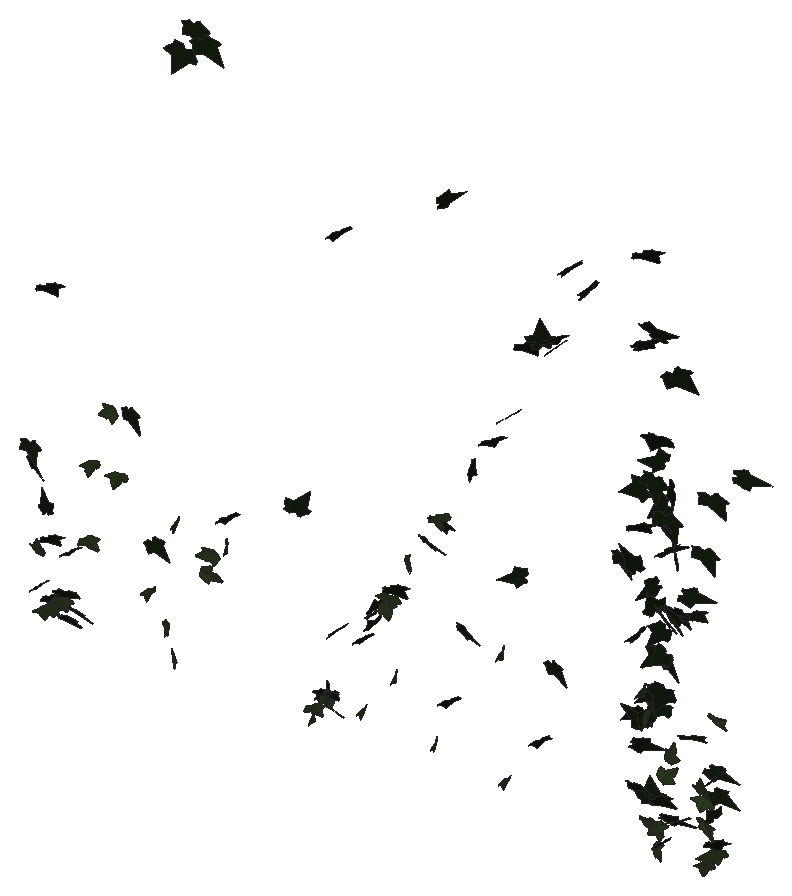
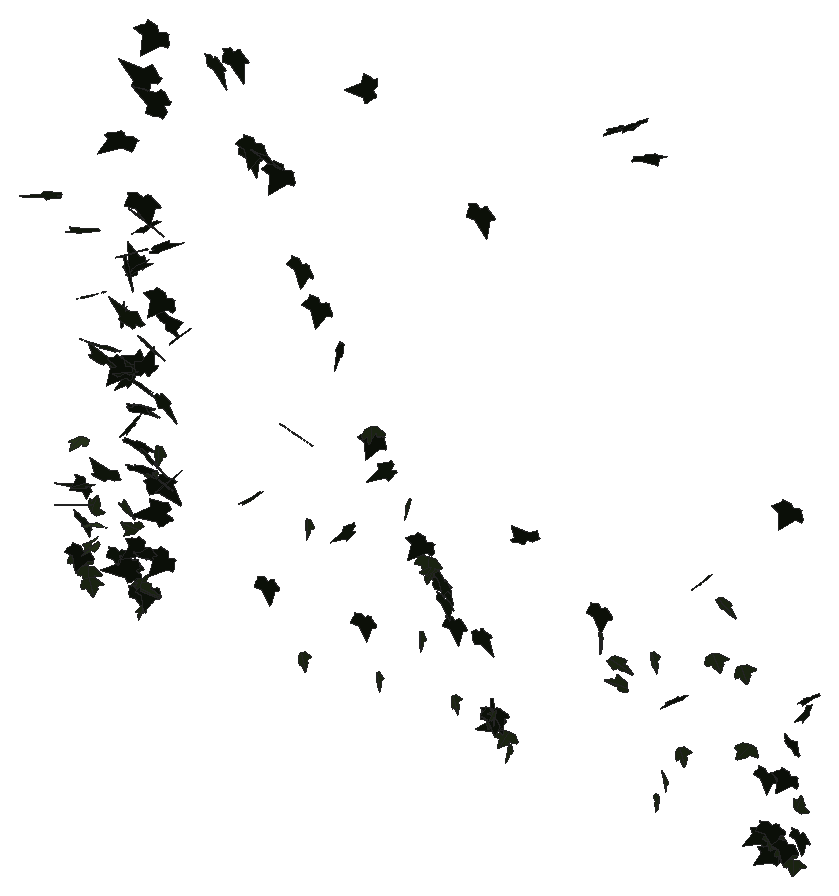
# SketchUp Ruby script. Lengths in inches.
U = 1.inch
M = Sketchup.active_model
def pt(a) = Geom::Point3d.new(a.map { |v| v * U })
def face(e, loops, mat)
  f = e.add_face(loops[0].map { |a| pt(a) })
  loops[1..].each { |l| e.add_face(l.map { |a| pt(a) }).erase! }
  f.material = f.back_material = mat if mat
  f
end
# faces: each face lists its corners as indices into pts; further lists are holes
def faces(e, pts, list, mat = nil) = list.each { |f| face(e, (f[0].is_a?(Array) ? f : [f]).map { |l| l.map { |i| pts[i] } }, mat) }
# xy, xz, yz: faces in a plane at the given z, y or x. An outline is a flat list of corners, or four numbers for a rectangle; further outlines are holes
def ring(l) = l.size == 4 ? [[l[0], l[1]], [l[2], l[1]], [l[2], l[3]], [l[0], l[3]]] : l.each_slice(2).to_a
def flat(e, list, mat, &to3) = list.each { |f| face(e, (f[0].is_a?(Array) ? f : [f]).map { |l| ring(l).map { |u, v| to3.(u, v) } }, mat) }
def xy(e, z, list, mat = nil) = flat(e, list, mat) { |x, y| [x, y, z] }
def xz(e, y, list, mat = nil) = flat(e, list, mat) { |x, z| [x, y, z] }
def yz(e, x, list, mat = nil) = flat(e, list, mat) { |y, z| [x, y, z] }
def lines(e, pts, list) = list.each { |a, b| e.add_line(pt(pts[a]), pt(pts[b])) }
# prism: a flat outline (further loops are holes) pulled along v
def prism(e, loops, v, mat = nil)
  f = face(e, loops, mat); d = Geom::Vector3d.new(v.map { |x| x * U })
  f.pushpull(f.normal.samedirection?(d) ? d.length : -d.length)
end
def box(e, o, s, mat = nil) = prism(e, [[o, [o[0] + s[0], o[1], o[2]], [o[0] + s[0], o[1] + s[1], o[2]], [o[0], o[1] + s[1], o[2]]]], [0, 0, s[2]], mat)
def at(x, y, z, deg = 0) = Geom::Transformation.translation(pt([x, y, z])) * Geom::Transformation.rotation(ORIGIN, Z_AXIS, deg.degrees)
def axes(o, x, y, z) = Geom::Transformation.new([*x, 0, *y, 0, *z, 0, *pt(o).to_a, 1])
def part(name) = M.definitions.add(name)
# library, detail: a bought-in or finely detailed component or shape, given as its bounding box
def library(name, o, s) = part(name).tap { |d| box(d.entities, o, s) }
def detail(e, o, s) = box(e.add_group.entities, o, s)
def put(e, d, t, mat = nil) = e.add_instance(d, t).tap { |i| i.material = mat if mat }
def group(e, t, mat = nil) = e.add_group.tap { |g| g.transformation = t; g.material = mat if mat }.entities
root = M.entities
M.materials.add("1026 AP 7946 SUNNY SIDE UP").color = [254, 231, 186]
M.materials.add("efeu1").color = [18, 25, 13]
M.materials.add("efeu2").color = [43, 57, 29]
c1 = part("ivyleaf_9")
p = [[1.54,2.16,1.25],[1.36,2.04,1.19],[-0.21,0.99,0.68],[-0.71,1.11,0.82],[-0.85,0.86,0.67],[-0.8,0.17,0.21],
  [-0.9,-0.01,0.1],[-0.67,-0.16,-0.02],[-0.08,-0.08,-0.05],[-0.03,-0.6,-0.4],[0.65,-0.88,-0.66],[0.83,-0.6,-0.49],
  [1.29,-0.42,-0.43],[1.8125,-0.07,-0.26],[1.21,0.44,0.15]]
faces(c1.entities,p,[[0,1,2,3,4,5,6,7,8,9,10,11,12,13,14]],"efeu1")
c2 = part("ivyleaf_10")
p = [[0,0.5,-0.03],[-0.0625,2.02,-0.43],[-0.19,2.01,-0.46],[-0.54,1.05,-0.29],[-0.52,0.625,-0.18],[-0.83,0.76,-0.28],
  [-1.16,0.64,-0.33],[-1.15,0.33,-0.24],[-0.77,-0.39,0.02],[-0.3,-0.51,0.16],[0.04,-0.48,0.23],[-0.02,2.01,-0.4375],
  [-0.06,2.01,-0.43],[0.04,-0.49,0.23],[0.67,-0.49,0.14],[1.38,0.36,-0.2],[1.375,0.51,-0.24],[0.81,0.65,-0.19],
  [0.62,0.59,-0.15],[0.6,1.09,-0.28],[0.5,1.23,-0.31]]
faces(c2.entities,p,[[0,1,2,3,4,5,6,7,8,9,10],[11,12,0,13,14,15,16,17,18,19,20]],"efeu2")
put(root,c1,axes([95.23,213.03,300.93],[-0.00357,-0.35074,-0.05937],[-0.00807,0.05091,-0.37476],[0.60158,-0.0014,-0.00538]),"1026 AP 7946 SUNNY SIDE UP")
put(root,c1,axes([95.375,212.96,300.02],[0.35506,-0.28,-0.0458],[-0.08733,0.01017,-0.37215],[0.47192,0.21255,-0.0344]),"1026 AP 7946 SUNNY SIDE UP")
put(root,c2,axes([95.79,213.17,294.47],[-0.49841,0.14012,-0.04801],[-0.04733,0.04941,0.34726],[0.2462,0.29316,-0.03043]),"1026 AP 7946 SUNNY SIDE UP")
put(root,c1,axes([96.05,212.75,292.63],[0.02986,0.32766,0.05959],[0.00064,0.05144,-0.35056],[-0.56301,0.01744,0.00277]),"1026 AP 7946 SUNNY SIDE UP")
put(root,c2,axes([96.24,213.05,291.09],[-0.39048,-0.21835,-0.01454],[0.02991,-0.00298,-0.33924],[0.3699,-0.23026,0.01208]),"1026 AP 7946 SUNNY SIDE UP")
put(root,c1,axes([96.5625,212.75,297.47],[0.19322,-0.04509,0.34792],[-0.15962,0.32567,0.08803],[-0.53463,-0.11353,0.09946]),"1026 AP 7946 SUNNY SIDE UP")
put(root,c1,axes([96.58,213.09,291.97],[0.30177,0.26789,-0.03101],[-0.00319,-0.03764,-0.34411],[-0.45807,0.17674,-0.01803]),"1026 AP 7946 SUNNY SIDE UP")
put(root,c1,axes([96.59,212.74,311.18],[0.44809,0.28118,0.02195],[0.0544,-0.00705,-0.41188],[-0.47507,0.26441,-0.02646]),"1026 AP 7946 SUNNY SIDE UP")
put(root,c2,axes([96.82,213.03,291.51],[-0.41117,-0.21127,-0.01285],[0.0413,-0.01387,-0.34312],[0.35661,-0.24199,0.02492]),"1026 AP 7946 SUNNY SIDE UP")
put(root,c1,axes([96.7,212.79,295.78],[0.40006,0.24658,0.05647],[0.08086,0.0229,-0.36431],[-0.41922,0.23973,-0.01637]),"1026 AP 7946 SUNNY SIDE UP")
put(root,c1,axes([97.14,212.86,291.79],[0.255,-0.06268,-0.30217],[-0.43607,0.11502,-0.17261],[0.22227,0.29756,0.00803]),"1026 AP 7946 SUNNY SIDE UP")
put(root,c2,axes([97.4,213.03,292.11],[-0.48203,-0.15261,-0.08488],[0.14499,-0.00375,-0.34998],[0.23021,-0.31719,0.0427]),"1026 AP 7946 SUNNY SIDE UP")
put(root,c1,axes([97.64,213.05,292.67],[0.31298,0.23347,-0.18068],[-0.20887,-0.11841,-0.31601],[-0.41029,0.23838,0.02305]),"1026 AP 7946 SUNNY SIDE UP")
put(root,c1,axes([97.52,213.03,291.13],[0.53819,0.0485,0.03464],[0.04617,0.03125,-0.34174],[-0.08686,0.31709,0.03295]),"1026 AP 7946 SUNNY SIDE UP")
put(root,c1,axes([98.125,212.8,295.44],[0.11966,0.33328,0.0627],[-0.00067,0.05547,-0.36371],[-0.5732,0.06951,0.01351]),"1026 AP 7946 SUNNY SIDE UP")
put(root,c1,axes([98.24,212.92,291.89],[0.55206,-0.05466,0.00803],[0.02378,0.04489,-0.36262],[0.08357,0.34831,0.05012]),"1026 AP 7946 SUNNY SIDE UP")
put(root,c2,axes([99.45,213.125,301.125],[-0.25583,-0.33417,0.09549],[0.01008,-0.10733,-0.37988],[0.546,-0.15459,0.05176]),"1026 AP 7946 SUNNY SIDE UP")
put(root,c2,axes([99.3,212.87,296.55],[-0.4094,-0.19196,-0.19442],[0.28625,0.06582,-0.32923],[0.31019,-0.3141,0.04722]),"1026 AP 7946 SUNNY SIDE UP")
put(root,c2,axes([100.64,213.28,304.64],[0.35432,-0.1591,-0.29218],[-0.40232,0.12445,-0.28151],[0.31358,0.33943,-0.03105]),"1026 AP 7946 SUNNY SIDE UP")
put(root,c2,axes([101.34,213.03,301.08],[-0.38148,-0.27016,0.12577],[-0.0591,-0.1304,-0.37036],[0.4634,-0.23903,0.0563]),"1026 AP 7946 SUNNY SIDE UP")
put(root,c1,axes([102.03,213.05,305.25],[0.18444,-0.37691,-0.04427],[-0.01339,0.04011,-0.4064],[0.59596,0.11754,0.00457]),"1026 AP 7946 SUNNY SIDE UP")
put(root,c2,axes([103.52,212.97,294.88],[-0.10461,-0.35823,0.02798],[-0.00227,-0.02942,-0.3755],[0.56514,-0.06643,0.00367]),"1026 AP 7946 SUNNY SIDE UP")
put(root,c1,axes([103.71,212.95,297.9],[0.17457,-0.29747,-0.21032],[0.02539,0.21579,-0.31624],[0.56524,0.08218,0.07916]),"1026 AP 7946 SUNNY SIDE UP")
put(root,c2,axes([104.65,212.95,293.1],[0.33264,-0.28479,-0.06698],[0.0119,0.08364,-0.36056],[0.45861,0.20439,0.05794]),"1026 AP 7946 SUNNY SIDE UP")
put(root,c2,axes([105.1,212.9,291.56],[-0.31441,0.29117,-0.04315],[-0.03658,-0.06809,-0.35946],[-0.46148,-0.19298,0.05789]),"1026 AP 7946 SUNNY SIDE UP")
put(root,c2,axes([105.3,212.97,299.71],[0.09906,-0.37566,-0.0326],[-0.00046,0.02987,-0.39221],[0.59251,0.06283,0.00514]),"1026 AP 7946 SUNNY SIDE UP")
put(root,c1,axes([105.63,213.23,328.52],[-0.45543,-0.35945,0.04426],[-0.01019,-0.05248,-0.47501],[0.56953,-0.28838,0.0269]),"1026 AP 7946 SUNNY SIDE UP")
put(root,c1,axes([106.27,213.29,330.24],[0.02494,-0.45731,-0.10528],[0.08561,0.10078,-0.46719],[0.73093,0.0038,0.05831]),"1026 AP 7946 SUNNY SIDE UP")
put(root,c1,axes([107.09,213.05,329.66],[0.0926,-0.40174,-0.24082],[0.19337,0.23852,-0.39283],[0.70295,-0.01269,0.13978]),"1026 AP 7946 SUNNY SIDE UP")
put(root,c2,axes([107.83,212.91,298.5625],[0.30268,-0.02002,-0.3376],[-0.5101,0.04598,-0.199],[0.07825,0.37717,0.00859]),"1026 AP 7946 SUNNY SIDE UP")
put(root,c2,axes([107.32,212.875,297.33],[0.07018,0.04826,0.38191],[0.57347,0.07517,-0.05492],[-0.12722,0.36547,-0.03687]),"1026 AP 7946 SUNNY SIDE UP")
put(root,c1,axes([108.75,212.9,301.2],[0.11336,0.38252,0.00033],[0.00233,-0.00216,-0.40101],[-0.60147,0.07209,-0.00149]),"1026 AP 7946 SUNNY SIDE UP")
put(root,c2,axes([108.82,212.82,299.59],[0.19604,-0.33424,-0.14877],[0.01982,0.15455,-0.36117],[0.57099,0.10939,0.06361]),"1026 AP 7946 SUNNY SIDE UP")
put(root,c1,axes([113.66,212.71,303.45],[-0.32406,-0.02014,0.35571],[0.51548,0.11716,0.20924],[-0.17392,0.38477,-0.04263]),"1026 AP 7946 SUNNY SIDE UP")
put(root,c2,axes([114.67,212.85,291.18],[0.0971,-0.28199,-0.21864],[0.03921,0.21682,-0.29024],[0.55206,0.0342,0.05907]),"1026 AP 7946 SUNNY SIDE UP")
put(root,c2,axes([114.82,212.82,291.8125],[-0.36896,-0.22627,-0.15802],[0.20942,0.07997,-0.33376],[0.37406,-0.26796,0.031]),"1026 AP 7946 SUNNY SIDE UP")
put(root,c1,axes([115.63,212.88,292.9],[0.24167,0.2189,-0.25071],[-0.24008,-0.19142,-0.27643],[-0.4569,0.21636,0.01264]),"1026 AP 7946 SUNNY SIDE UP")
put(root,c1,axes([115.58,212.84,292.79],[0.14638,0.35072,-0.0142],[-0.006,-0.01531,-0.37391],[-0.552,0.09317,0.0003]),"1026 AP 7946 SUNNY SIDE UP")
put(root,c2,axes([115.59,212.85,292.84],[-0.11215,0.3515,0.01797],[-0.085,0.00463,-0.36556],[-0.54666,-0.07283,0.05315]),"1026 AP 7946 SUNNY SIDE UP")
put(root,c1,axes([115.84,212.77,293.3],[0.16952,-0.09094,-0.34698],[-0.49821,0.12074,-0.13757],[0.2277,0.33187,-0.04269]),"1026 AP 7946 SUNNY SIDE UP")
put(root,c2,axes([115.58,212.85,292.66],[0.24726,0.29598,0.14444],[0.01136,0.15055,-0.33894],[-0.51373,0.14579,0.06203]),"1026 AP 7946 SUNNY SIDE UP")
put(root,c1,axes([115.31,212.87,292.26],[0.48861,-0.17513,0.05272],[0.11765,0.02805,-0.36197],[0.26213,0.31384,0.06419]),"1026 AP 7946 SUNNY SIDE UP")
put(root,c1,axes([116.48,212.89,297.1],[-0.16077,0.33809,-0.12939],[0.01209,-0.13046,-0.36345],[-0.56804,-0.09847,0.02888]),"1026 AP 7946 SUNNY SIDE UP")
put(root,c1,axes([116.51,212.83,321.45],[0.03351,0.44655,-0.06141],[-0.00041,-0.06221,-0.46091],[-0.70892,0.02114,-0.00264]),"1026 AP 7946 SUNNY SIDE UP")
put(root,c1,axes([118.16,212.81,297.16],[0.03937,0.37771,-0.00849],[0.00029,-0.01042,-0.39003],[-0.59413,0.02503,-0.00075]),"1026 AP 7946 SUNNY SIDE UP")
put(root,c2,axes([118.11,212.9375,292.76],[0.03919,-0.35756,-0.00565],[0.00814,0.00382,-0.36918],[0.56219,0.02487,0.00574]),"1026 AP 7946 SUNNY SIDE UP")
put(root,c1,axes([118.82,212.83,298.2],[-0.06508,0.33985,0.17693],[-0.06461,0.16581,-0.35121],[-0.59387,-0.05528,0.01882]),"1026 AP 7946 SUNNY SIDE UP")
put(root,c1,axes([118.9375,212.77,299.23],[0.04365,0.2671,0.28509],[-0.03407,0.27659,-0.27267],[-0.60209,0.00372,0.0361]),"1026 AP 7946 SUNNY SIDE UP")
put(root,c1,axes([119.13,212.78,299.11],[-0.17113,0.36333,-0.02991],[-0.04093,-0.04011,-0.38917],[-0.57193,-0.10585,0.0368]),"1026 AP 7946 SUNNY SIDE UP")
put(root,c2,axes([119.63,212.82,299.62],[0.19033,0.35589,0.09671],[0.00542,0.09561,-0.38572],[-0.57791,0.11811,0.02824]),"1026 AP 7946 SUNNY SIDE UP")
put(root,c2,axes([119.81,212.97,300.17],[-0.58691,-0.09079,0.01008],[-0.00338,-0.03459,-0.39447],[0.14364,-0.37179,0.03191]),"1026 AP 7946 SUNNY SIDE UP")
put(root,c2,axes([120.31,212.87,295.63],[0.08062,-0.32197,-0.17951],[0.00294,0.17434,-0.33379],[0.57428,0.04431,0.02691]),"1026 AP 7946 SUNNY SIDE UP")
put(root,c1,axes([120.18,212.74,300.98],[0.47973,0.23969,0.04964],[0.09556,-0.00195,-0.39771],[-0.37193,0.30866,-0.03816]),"1026 AP 7946 SUNNY SIDE UP")
put(root,c2,axes([121.21,212.75,302.91],[-0.21852,0.30821,0.21585],[-0.17319,0.17771,-0.34643],[-0.55821,-0.17579,0.02298]),"1026 AP 7946 SUNNY SIDE UP")
put(root,c1,axes([122.24,212.95,304.56],[0.59073,-0.10892,-0.08336],[-0.06724,0.12925,-0.38597],[0.20187,0.36178,0.11538]),"1026 AP 7946 SUNNY SIDE UP")
put(root,c2,axes([122.98,212.98,292.41],[0.0995,-0.33778,-0.10226],[-0.00251,0.09863,-0.35307],[0.55273,0.06125,0.01681]),"1026 AP 7946 SUNNY SIDE UP")
put(root,c1,axes([123.16,212.94,306.06],[0.56153,0.10197,-0.16151],[-0.25262,-0.00812,-0.3811],[-0.15202,0.39016,0.03671]),"1026 AP 7946 SUNNY SIDE UP")
put(root,c2,axes([123.42,212.96,306.35],[-0.30143,-0.35517,-0.01126],[0.07215,-0.01471,-0.413],[0.55396,-0.19134,0.04766]),"1026 AP 7946 SUNNY SIDE UP")
put(root,c1,axes([123.95,212.88,295.33],[0.09992,0.36378,-0.03255],[-0.01538,-0.03246,-0.38061],[-0.57425,0.06417,0.00453]),"1026 AP 7946 SUNNY SIDE UP")
put(root,c1,axes([123.63,212.69,325.82],[0.17104,0.11909,0.45524],[0.49559,0.30888,-0.16413],[-0.52037,0.33331,-0.00668]),"1026 AP 7946 SUNNY SIDE UP")
put(root,c1,axes([124.82,212.85,300.09],[0.49462,-0.19341,-0.11816],[-0.07715,0.1316,-0.37001],[0.34416,0.30747,0.08687]),"1026 AP 7946 SUNNY SIDE UP")
put(root,c1,axes([125.66,212.6875,310.32],[0.10953,-0.10368,-0.41477],[-0.47342,0.26807,-0.1234],[0.44951,0.30759,-0.02889]),"1026 AP 7946 SUNNY SIDE UP")
put(root,c1,axes([126.9,212.76,312.35],[0.24124,0.39837,0.03274],[0.00593,0.03017,-0.43954],[-0.62808,0.15329,0.00843]),"1026 AP 7946 SUNNY SIDE UP")
put(root,c2,axes([127.5625,212.9,299.58],[0.05429,-0.34251,-0.17661],[0.01871,0.17106,-0.35262],[0.6006,0.02563,0.02695]),"1026 AP 7946 SUNNY SIDE UP")
put(root,c2,axes([127.84,212.99,291.84],[-0.02811,-0.35359,-0.01754],[-0.00236,0.01511,-0.36464],[0.55649,-0.0178,-0.00243]),"1026 AP 7946 SUNNY SIDE UP")
put(root,c1,axes([128.08,212.75,314.18],[0.10329,0.40782,0.1379],[-0.02313,0.13515,-0.42329],[-0.67339,0.05791,0.03569]),"1026 AP 7946 SUNNY SIDE UP")
put(root,c1,axes([128.95,212.94,304.63],[-0.53728,0.18692,0.09214],[-0.18695,-0.03797,-0.39105],[-0.26598,-0.35089,0.08874]),"1026 AP 7946 SUNNY SIDE UP")
put(root,c1,axes([129.34,212.65,319.09],[0.46967,0.33078,0.03033],[0.05199,0.00725,-0.45865],[-0.51933,0.29987,-0.01848]),"1026 AP 7946 SUNNY SIDE UP")
put(root,c1,axes([130.26,212.78,295.17],[0.07678,0.3673,-0.04204],[0.00918,-0.04403,-0.38179],[-0.58139,0.04781,-0.01158]),"1026 AP 7946 SUNNY SIDE UP")
put(root,c1,axes([130.42,212.8,319.49],[-0.66849,0.13416,-0.0313],[-0.02594,0.05075,0.45739],[0.21501,0.42325,-0.04216]),"1026 AP 7946 SUNNY SIDE UP")
put(root,c1,axes([131.13,212.71,320.03],[0.25982,0.41392,0.07602],[0.00718,0.075,-0.45808],[-0.66044,0.16365,0.02493]),"1026 AP 7946 SUNNY SIDE UP")
put(root,c1,axes([131.42,212.74,319.65],[-0.06155,0.44642,0.03891],[-0.00919,0.03486,-0.46145],[-0.70408,-0.03948,0.00262]),"1026 AP 7946 SUNNY SIDE UP")
put(root,c1,axes([130.96,212.99,299.92],[0.23087,-0.34764,-0.06133],[0.03864,0.0723,-0.38489],[0.55272,0.14015,0.05252]),"1026 AP 7946 SUNNY SIDE UP")
put(root,c1,axes([132.37,212.79,324.86],[-0.05791,0.45536,-0.07268],[0.00979,-0.07287,-0.47107],[-0.72513,-0.03735,-0.00056]),"1026 AP 7946 SUNNY SIDE UP")
put(root,c1,axes([133.75,212.7,323.96],[-0.23058,0.43487,0.05846],[-0.02603,0.0517,-0.47248],[-0.68861,-0.14757,-0.00172]),"1026 AP 7946 SUNNY SIDE UP")
put(root,c1,axes([135.23,213.5,307.99],[0.16161,-0.40448,-0.08323],[-0.03547,0.07525,-0.42948],[0.6469,0.10518,-0.00276]),"1026 AP 7946 SUNNY SIDE UP")
put(root,c1,axes([135.62,214.93,325.91],[0.50457,0.34979,0.07355],[0.07726,0.04911,-0.48872],[-0.55538,0.32462,-0.00117]),"1026 AP 7946 SUNNY SIDE UP")
put(root,c1,axes([136.09,213.75,309.9],[0.46235,0.29894,0.09312],[0.07653,0.07642,-0.43111],[-0.4843,0.29747,0.02078]),"1026 AP 7946 SUNNY SIDE UP")
put(root,c1,axes([136.65,212.9375,307.91],[0.05245,0.00757,0.4471],[-0.39198,0.35661,0.01542],[-0.55865,-0.24951,0.03116]),"1026 AP 7946 SUNNY SIDE UP")
put(root,c1,axes([136.68,213.29,303.73],[-0.30823,0.35317,-0.04868],[0.00697,-0.05379,-0.41582],[-0.56067,-0.19483,0.02159]),"1026 AP 7946 SUNNY SIDE UP")
put(root,c1,axes([136.78,213.38,299],[0.022,0.25585,-0.36837],[-0.28031,-0.32524,-0.24783],[-0.634,0.15268,0.0968]),"1026 AP 7946 SUNNY SIDE UP")
put(root,c1,axes([136.76,213.59,312.46],[-0.35744,-0.11889,0.36831],[-0.38583,-0.27116,-0.25472],[0.4509,-0.32627,0.07401]),"1026 AP 7946 SUNNY SIDE UP")
put(root,c1,axes([136.73,213.25,298.5],[-0.06289,-0.43977,-0.01343],[0.07831,-0.01504,0.45179],[-0.68724,0.03853,0.05271]),"1026 AP 7946 SUNNY SIDE UP")
put(root,c1,axes([136.26,213.74,320.97],[0.34738,0.4058,-0.12358],[0.0585,0.11878,0.47608],[0.66384,-0.22282,0.02271]),"1026 AP 7946 SUNNY SIDE UP")
put(root,c1,axes([136.54,213.04,294.5],[0.67802,0.00173,-0.0792],[-0.12021,-0.03794,-0.4428],[-0.01314,0.43635,-0.03562]),"1026 AP 7946 SUNNY SIDE UP")
put(root,c1,axes([137.12,214.23,315.48],[0.37514,0.25486,-0.28294],[-0.30708,-0.19529,-0.36071],[-0.50474,0.30823,0.00916]),"1026 AP 7946 SUNNY SIDE UP")
put(root,c2,axes([137.04,213.06,300.52],[-0.03011,-0.3483,-0.19828],[0.00545,0.19056,-0.35819],[0.62421,-0.01846,-0.00643]),"1026 AP 7946 SUNNY SIDE UP")
put(root,c1,axes([137.4375,213.04,298.78],[-0.19039,0.19392,0.3265],[-0.37043,0.21622,-0.22855],[-0.44986,-0.26011,0.05001]),"1026 AP 7946 SUNNY SIDE UP")
put(root,c1,axes([136.62,213.08,297.04],[0.45704,0.12549,0.31992],[0.48137,0.06497,-0.32259],[-0.21111,0.41983,-0.04298]),"1026 AP 7946 SUNNY SIDE UP")
put(root,c1,axes([137.69,213.96,314.28],[-0.44825,0.29613,0.16379],[-0.26345,0.05306,-0.41538],[-0.45672,-0.32124,0.07885]),"1026 AP 7946 SUNNY SIDE UP")
put(root,c1,axes([137.55,213.52,300.36],[-0.55947,0.23769,-0.05917],[0.04949,-0.05845,-0.44001],[-0.38182,-0.35586,0.02968]),"1026 AP 7946 SUNNY SIDE UP")
put(root,c1,axes([137.58,215,312.02],[0.10982,-0.08164,-0.48398],[-0.70628,0.14672,-0.0943],[0.24952,0.45124,-0.0539]),"1026 AP 7946 SUNNY SIDE UP")
put(root,c1,axes([137.53,213.59,306.84],[-0.59889,0.12445,-0.11422],[0.1293,-0.10221,-0.40723],[-0.22882,-0.3835,0.06883]),"1026 AP 7946 SUNNY SIDE UP")
put(root,c2,axes([137.77,213.2,292.27],[-0.0827,-0.00499,-0.41178],[-0.53418,0.21297,0.04456],[0.33117,0.34228,-0.03095]),"1026 AP 7946 SUNNY SIDE UP")
put(root,c1,axes([137.4,213.68,305.25],[0.19238,0.23464,0.37898],[-0.48936,-0.21898,0.25015],[0.47836,-0.31838,0.10349]),"1026 AP 7946 SUNNY SIDE UP")
put(root,c2,axes([137.36,213.03,299.01],[0.0398,0.3289,0.21841],[-0.11009,0.21099,-0.33028],[-0.60376,-0.01679,0.07462]),"1026 AP 7946 SUNNY SIDE UP")
put(root,c1,axes([137.45,213.13,292.38],[0.50584,0.09165,-0.23989],[-0.39163,0.07314,-0.32367],[-0.04535,0.39065,0.11937]),"1026 AP 7946 SUNNY SIDE UP")
put(root,c1,axes([137.53,214.46,311.35],[-0.28119,-0.28221,0.33953],[-0.23186,-0.29757,-0.34499],[0.64369,-0.23047,0.02405]),"1026 AP 7946 SUNNY SIDE UP")
put(root,c1,axes([137.78,213.02,294.1],[-0.58589,-0.05168,0.13751],[0.19852,0.05845,0.38587],[-0.10696,0.39156,-0.03707]),"1026 AP 7946 SUNNY SIDE UP")
put(root,c1,axes([137.07,213.8125,322.08],[0.12279,-0.14221,0.45949],[0.63379,-0.21113,-0.14302],[0.37678,0.40148,0.09084]),"1026 AP 7946 SUNNY SIDE UP")
put(root,c1,axes([137.87,213.78,299.59],[-0.62464,-0.15036,0.02596],[-0.01515,-0.0478,-0.4358],[0.23947,-0.39523,0.04015]),"1026 AP 7946 SUNNY SIDE UP")
put(root,c1,axes([137.54,213.49,313.41],[-0.09827,-0.45766,0.02587],[0.00361,-0.02827,-0.47597],[0.72093,-0.06224,0.00591]),"1026 AP 7946 SUNNY SIDE UP")
put(root,c1,axes([138.125,213.53,302.8125],[-0.55684,-0.14509,0.12264],[-0.15304,-0.07742,-0.39323],[0.25327,-0.36577,0.03202]),"1026 AP 7946 SUNNY SIDE UP")
put(root,c1,axes([138.12,213.51,302.9],[-0.59613,-0.12281,0.048],[-0.05059,-0.05332,-0.40873],[0.20065,-0.37832,0.03954]),"1026 AP 7946 SUNNY SIDE UP")
put(root,c1,axes([138.07,213.6,304.32],[-0.61696,-0.02119,-0.10714],[0.1667,-0.07751,-0.3967],[0.00038,-0.39841,0.08045]),"1026 AP 7946 SUNNY SIDE UP")
put(root,c1,axes([137.4,214.62,308.45],[0.25044,-0.41009,0.14738],[0.67051,0.1779,0.03673],[-0.13599,0.1219,0.45253]),"1026 AP 7946 SUNNY SIDE UP")
put(root,c1,axes([137.67,215.06,319.18],[-0.02863,-0.16962,-0.46481],[0.1364,0.442,-0.17258],[0.74411,-0.08755,0.01375]),"1026 AP 7946 SUNNY SIDE UP")
put(root,c1,axes([137.73,214.12,302.29],[0.35597,-0.35846,-0.12438],[-0.12622,0.08955,-0.43579],[0.58017,0.23942,-0.01849]),"1026 AP 7946 SUNNY SIDE UP")
put(root,c2,axes([138.02,213.03,291.2],[-0.06137,0.37731,0.06991],[-0.02936,0.06411,-0.39021],[-0.6015,-0.04163,0.01191]),"1026 AP 7946 SUNNY SIDE UP")
put(root,c1,axes([137.82,214.22,305.1],[0.51546,-0.29235,-0.10915],[-0.15799,0.04357,-0.45093],[0.46178,0.34124,-0.03245]),"1026 AP 7946 SUNNY SIDE UP")
put(root,c1,axes([138.24,213.44,300.72],[-0.60539,-0.16915,-0.13719],[0.2233,0.00292,-0.42989],[0.25316,-0.40707,0.05113]),"1026 AP 7946 SUNNY SIDE UP")
put(root,c2,axes([138.16,212.96,292.65],[0.10966,0.38012,-0.01865],[0.00388,-0.02105,-0.3982],[-0.59853,0.06951,-0.006]),"1026 AP 7946 SUNNY SIDE UP")
put(root,c1,axes([138.44,214.26,308.16],[0.02296,-0.22239,0.40269],[0.05094,0.39186,0.22999],[-0.70704,0.02101,0.02965]),"1026 AP 7946 SUNNY SIDE UP")
put(root,c1,axes([138.59,212.83,291.83],[-0.08783,0.34786,-0.07356],[0.0064,-0.07365,-0.3633],[-0.55897,-0.0555,0.0074]),"1026 AP 7946 SUNNY SIDE UP")
put(root,c1,axes([138,213.49,305.25],[0.27642,-0.26124,0.29884],[0.20506,-0.26228,-0.32463],[0.5804,0.21708,-0.02763]),"1026 AP 7946 SUNNY SIDE UP")
put(root,c1,axes([138.29,212.74,294.39],[0.45577,0.19716,0.12359],[0.1927,0.02962,-0.35836],[-0.30644,0.31187,-0.04153]),"1026 AP 7946 SUNNY SIDE UP")
put(root,c1,axes([138.23,214.26,305.15],[-0.17424,-0.36117,0.23179],[0.32607,-0.2506,-0.30788],[0.58621,0.03204,0.24015]),"1026 AP 7946 SUNNY SIDE UP")
put(root,c1,axes([138.19,213.32,310.77],[0.57265,-0.17888,-0.22512],[0.35055,-0.03412,0.41326],[-0.27056,-0.42282,0.05896]),"1026 AP 7946 SUNNY SIDE UP")
put(root,c2,axes([138.5,213.56,296.64],[0.54526,-0.20069,0.02839],[0.001,0.05794,0.40982],[-0.31877,-0.34309,0.04985]),"1026 AP 7946 SUNNY SIDE UP")
put(root,c1,axes([138.42,214.14,305.37],[0.68262,0.0292,-0.08844],[-0.13032,-0.04451,-0.44678],[-0.05844,0.44032,-0.03668]),"1026 AP 7946 SUNNY SIDE UP")
put(root,c2,axes([138.42,213.18,295.57],[0.26621,0.15308,-0.34129],[0.33972,0.25347,0.23527],[0.46402,-0.27339,0.02355]),"1026 AP 7946 SUNNY SIDE UP")
put(root,c1,axes([138.53,213.27,311.47],[-0.03673,-0.47148,-0.04341],[0.17412,0.03296,-0.47307],[0.72328,-0.03188,0.11168]),"1026 AP 7946 SUNNY SIDE UP")
put(root,c1,axes([139.08,212.73,293.24],[0.09807,0.3591,-0.01093],[-0.15664,0.00494,-0.36135],[-0.54285,0.06345,0.10229]),"1026 AP 7946 SUNNY SIDE UP")
put(root,c1,axes([138.52,213.1875,293.15],[0.54454,-0.02816,0.25027],[0.38453,0.05542,-0.35197],[-0.01425,0.41947,0.06581]),"1026 AP 7946 SUNNY SIDE UP")
put(root,c1,axes([138.89,214.51,306.33],[0.46772,-0.27129,-0.09736],[0.38369,0.3098,-0.12521],[0.2369,0.03387,0.39501]),"1026 AP 7946 SUNNY SIDE UP")
put(root,c1,axes([139.79,212.8,293.55],[0.05961,0.36273,-0.01541],[-0.06321,-0.01282,-0.37368],[-0.56748,0.03953,0.04001]),"1026 AP 7946 SUNNY SIDE UP")
put(root,c1,axes([139.39,214.4,305.38],[0.01671,-0.40985,-0.01695],[0.62931,0.01345,-0.09164],[0.1406,-0.01148,0.41222]),"1026 AP 7946 SUNNY SIDE UP")
put(root,c1,axes([139.76,213.75,298.32],[0.01549,-0.36687,0.11803],[0.57451,-0.02785,-0.12219],[0.19071,0.11371,0.35852]),"1026 AP 7946 SUNNY SIDE UP")
put(root,c1,axes([139.91,214.79,309.21],[-0.01995,-0.43752,-0.02061],[0.19962,0.0131,-0.43162],[0.65893,-0.01721,0.13014]),"1026 AP 7946 SUNNY SIDE UP")
put(root,c1,axes([140.41,214.78,312.72],[-0.02507,-0.44894,-0.03817],[0.38531,0.02032,-0.38882],[0.59397,-0.03213,0.25061]),"1026 AP 7946 SUNNY SIDE UP")
put(root,c2,axes([141.01,213.43,294.94],[-0.54396,-0.09866,0.0979],[0.15238,-0.35885,-0.02233],[0.15309,0.00663,0.37008]),"1026 AP 7946 SUNNY SIDE UP")
put(root,c2,axes([141.18,213.07,295.7],[-0.53044,0.1612,-0.05366],[-0.05037,0.05533,0.38373],[0.26203,0.33697,-0.03486]),"1026 AP 7946 SUNNY SIDE UP")
put(root,c2,axes([141.03,213.15,293.68],[0.36097,-0.2521,-0.18777],[0.29372,0.29192,-0.17326],[0.38951,0.0135,0.30466]),"1026 AP 7946 SUNNY SIDE UP")
put(root,c2,axes([141.48,213.04,291.37],[-0.34867,-0.28063,0.0609],[-0.03186,-0.06122,-0.36814],[0.45034,-0.2216,0.0211]),"1026 AP 7946 SUNNY SIDE UP")
put(root,c2,axes([141.46,213.76,299.88],[0.54163,-0.10721,-0.17211],[0.13157,0.38155,-0.07255],[0.28217,0.02788,0.36421]),"1026 AP 7946 SUNNY SIDE UP")
put(root,c2,axes([141.67,212.95,291.96],[-0.41558,-0.25083,-0.01517],[0.03183,-0.00202,-0.37505],[0.39367,-0.26463,0.01431]),"1026 AP 7946 SUNNY SIDE UP")
put(root,c2,axes([141.36,213.1,293.66],[-0.11385,-0.30716,0.20626],[0.45857,-0.17331,-0.16484],[0.35189,0.12647,0.28155]),"1026 AP 7946 SUNNY SIDE UP")
put(root,c1,axes([142.18,212.76,294.65],[-0.07489,0.30427,0.21589],[-0.14543,0.19298,-0.31177],[-0.56085,-0.09067,0.05202]),"1026 AP 7946 SUNNY SIDE UP")
put(root,c1,axes([141.96,212.88,296.8],[-0.18141,0.22849,-0.28086],[-0.16197,0.2543,0.2647],[0.537,0.15389,-0.01504]),"1026 AP 7946 SUNNY SIDE UP")
put(root,c1,axes([142.02,212.98,292.9375],[0.32117,0.30794,-0.03539],[-0.00339,-0.04182,-0.3803],[-0.48752,0.20316,-0.02067]),"1026 AP 7946 SUNNY SIDE UP")
put(root,c1,axes([141.56,213.4,297.03],[0.375,-0.30548,-0.09769],[0.30587,0.23111,-0.26652],[0.39823,0.11015,0.2967]),"1026 AP 7946 SUNNY SIDE UP")
put(root,c2,axes([142.28,212.93,292.43],[-0.4376,-0.24271,-0.01333],[0.04396,-0.01451,-0.3793],[0.37953,-0.27816,0.02855]),"1026 AP 7946 SUNNY SIDE UP")
put(root,c1,axes([141.89,213.28,295.8],[0.25247,-0.30045,-0.17998],[0.2649,0.23424,-0.25664],[0.47645,0.02897,0.23806]),"1026 AP 7946 SUNNY SIDE UP")
put(root,c1,axes([142.03,215.15,314.37],[0.6144,-0.18737,-0.12015],[0.15085,0.35684,-0.25976],[0.31155,0.19673,0.36272]),"1026 AP 7946 SUNNY SIDE UP")
